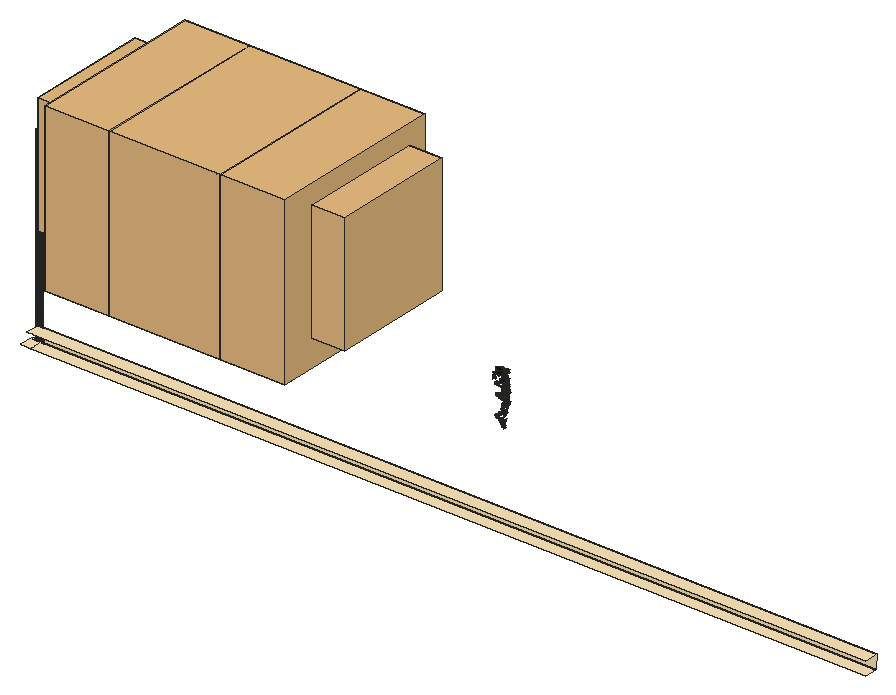
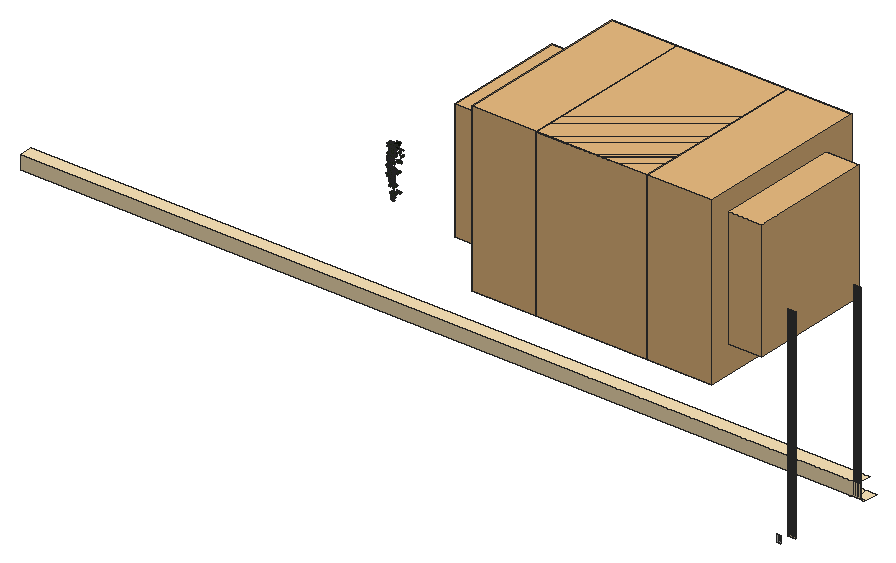
# SketchUp Ruby script. Lengths in inches.
U = 1.inch
M = Sketchup.active_model
def pt(a) = Geom::Point3d.new(a.map { |v| v * U })
def face(e, loops, mat)
  f = e.add_face(loops[0].map { |a| pt(a) })
  loops[1..].each { |l| e.add_face(l.map { |a| pt(a) }).erase! }
  f.material = f.back_material = mat if mat
  f
end
# faces: each face lists its corners as indices into pts; further lists are holes
def faces(e, pts, list, mat = nil) = list.each { |f| face(e, (f[0].is_a?(Array) ? f : [f]).map { |l| l.map { |i| pts[i] } }, mat) }
# xy, xz, yz: faces in a plane at the given z, y or x. An outline is a flat list of corners, or four numbers for a rectangle; further outlines are holes
def ring(l) = l.size == 4 ? [[l[0], l[1]], [l[2], l[1]], [l[2], l[3]], [l[0], l[3]]] : l.each_slice(2).to_a
def flat(e, list, mat, &to3) = list.each { |f| face(e, (f[0].is_a?(Array) ? f : [f]).map { |l| ring(l).map { |u, v| to3.(u, v) } }, mat) }
def xy(e, z, list, mat = nil) = flat(e, list, mat) { |x, y| [x, y, z] }
def xz(e, y, list, mat = nil) = flat(e, list, mat) { |x, z| [x, y, z] }
def yz(e, x, list, mat = nil) = flat(e, list, mat) { |y, z| [x, y, z] }
def lines(e, pts, list) = list.each { |a, b| e.add_line(pt(pts[a]), pt(pts[b])) }
# prism: a flat outline (further loops are holes) pulled along v
def prism(e, loops, v, mat = nil)
  f = face(e, loops, mat); d = Geom::Vector3d.new(v.map { |x| x * U })
  f.pushpull(f.normal.samedirection?(d) ? d.length : -d.length)
end
def box(e, o, s, mat = nil) = prism(e, [[o, [o[0] + s[0], o[1], o[2]], [o[0] + s[0], o[1] + s[1], o[2]], [o[0], o[1] + s[1], o[2]]]], [0, 0, s[2]], mat)
def at(x, y, z, deg = 0) = Geom::Transformation.translation(pt([x, y, z])) * Geom::Transformation.rotation(ORIGIN, Z_AXIS, deg.degrees)
def axes(o, x, y, z) = Geom::Transformation.new([*x, 0, *y, 0, *z, 0, *pt(o).to_a, 1])
def part(name) = M.definitions.add(name)
# library, detail: a bought-in or finely detailed component or shape, given as its bounding box
def library(name, o, s) = part(name).tap { |d| box(d.entities, o, s) }
def detail(e, o, s) = box(e.add_group.entities, o, s)
def put(e, d, t, mat = nil) = e.add_instance(d, t).tap { |i| i.material = mat if mat }
def group(e, t, mat = nil) = e.add_group.tap { |g| g.transformation = t; g.material = mat if mat }.entities
root = M.entities
M.materials.add("1026 AP 7946 SUNNY SIDE UP").color = [254, 231, 186]
M.materials.add("efeu1").color = [18, 25, 13]
M.materials.add("efeu2").color = [43, 57, 29]
c1 = library("Plante \#58",[-0.43,-1.58,0],[20.84,18.06,17.59])
c2 = library("Plant+Philodendron+Scandens",[-5.75,-7.35,0],[25.95,25.95,24.43])
c3 = part("ivyleaf_10")
p = [[0,0.5,-0.03],[-0.0625,2.02,-0.43],[-0.19,2.01,-0.46],[-0.54,1.05,-0.29],[-0.52,0.625,-0.18],[-0.83,0.76,-0.28],
  [-1.16,0.64,-0.33],[-1.15,0.33,-0.24],[-0.77,-0.39,0.02],[-0.3,-0.51,0.16],[0.04,-0.48,0.23],[-0.02,2.01,-0.4375],
  [-0.06,2.01,-0.43],[0.04,-0.49,0.23],[0.67,-0.49,0.14],[1.38,0.36,-0.2],[1.375,0.51,-0.24],[0.81,0.65,-0.19],
  [0.62,0.59,-0.15],[0.6,1.09,-0.28],[0.5,1.23,-0.31]]
faces(c3.entities,p,[[0,1,2,3,4,5,6,7,8,9,10],[11,12,0,13,14,15,16,17,18,19,20]],"efeu2")
c4 = part("ivyleaf_9")
p = [[1.54,2.16,1.25],[1.36,2.04,1.19],[-0.21,0.99,0.68],[-0.71,1.11,0.82],[-0.85,0.86,0.67],[-0.8,0.17,0.21],
  [-0.9,-0.01,0.1],[-0.67,-0.16,-0.02],[-0.08,-0.08,-0.05],[-0.03,-0.6,-0.4],[0.65,-0.88,-0.66],[0.83,-0.6,-0.49],
  [1.29,-0.42,-0.43],[1.8125,-0.07,-0.26],[1.21,0.44,0.15]]
faces(c4.entities,p,[[0,1,2,3,4,5,6,7,8,9,10,11,12,13,14]],"efeu1")
xy(root,246,[[152.978,213.099,30,213.101,29.751,213.101,29.492,213.104,29.53,215.005,29.675,215.002,29.749,215.001,29.764,215.001,30,215,153,215],[29.492,213.104,29.19,213.112,28.983,213.119,28.649,213.135,28.378,213.15,28.108,213.169,27.896,213.185,28.055,215.079,28.117,215.074,28.184,215.069,28.242,215.064,28.294,215.061,28.352,215.057,28.428,215.052,28.493,215.047,28.538,215.045,28.587,215.042,28.673,215.037,28.744,215.033,28.781,215.031,28.822,215.029,28.918,215.025,28.995,215.021,29.025,215.02,29.058,215.019,29.165,215.015,29.246,215.012,29.269,215.011,29.293,215.01,29.416,215.007,29.497,215.005,29.53,215.005],[153,215,30,215.001,29.749,215.001,29.675,215.002,29.53,215.005,29.532,215.104,29.766,215.101,30,215.101,153,215.099],[30,215,29.764,215.001,29.749,215.001,29.675,215.002,29.53,215.005,29.532,215.104,29.766,215.101,30,215.101,153,215.099,153.002,215.099,153,215],[30,215,30,215.001,29.764,215.001],
  [30,215,153,215,30,215.001],[29.497,215.005,29.416,215.007,29.293,215.01,29.269,215.011,29.246,215.012,29.165,215.015,29.058,215.019,29.025,215.02,28.995,215.021,28.918,215.025,28.822,215.029,28.781,215.031,28.744,215.033,28.673,215.037,28.587,215.042,28.538,215.045,28.493,215.047,28.428,215.052,28.352,215.057,28.294,215.061,28.242,215.064,28.184,215.069,28.117,215.074,28.055,215.079,28.064,215.178,28.254,215.163,28.503,215.146,28.752,215.132,29.064,215.118,29.251,215.111,29.532,215.104,29.53,215.005],[29.764,227.001,29.647,227.004,29.749,227.003,29.913,227.001]],"1026 AP 7946 SUNNY SIDE UP")
xy(root,248,[[152.981,213.1,153.004,215.1,30,215.101,29.766,215.101,29.532,215.104,29.251,215.111,29.064,215.118,28.983,213.12,29.19,213.112,29.492,213.105,29.751,213.101,30,213.101]],"1026 AP 7946 SUNNY SIDE UP")
xz(root,215.001,[[29.749,246,29.756,274],[29.756,246,29.764,274]],"1026 AP 7946 SUNNY SIDE UP")
xz(root,215.005,[[29.497,246,29.513,274],[29.513,246,29.529,274]],"1026 AP 7946 SUNNY SIDE UP")
xz(root,227.001,[[29.764,246,29.809,249],[29.809,246,29.913,249]],"1026 AP 7946 SUNNY SIDE UP")
p = [[28.744,215.033,246],[28.781,215.031,246],[28.781,215.031,274],[28.744,215.033,274],[28.822,215.029,246],[28.822,215.029,274],
  [28.918,215.025,246],[28.918,215.025,274],[28.995,215.021,246],[28.995,215.021,274],[29.025,215.02,246],[29.025,215.02,274],
  [29.058,215.019,246],[29.058,215.019,274],[29.165,215.015,246],[29.165,215.015,274],[29.246,215.012,246],[29.246,215.012,274],
  [29.269,215.011,246],[29.269,215.011,274],[29.293,215.01,246],[29.293,215.01,274],[29.416,215.007,246],[29.416,215.007,274],
  [29.497,215.005,246],[29.497,215.005,274],[29.53,215.005,246],[29.675,215.002,246],[29.675,215.002,274],[29.529,215.005,274],
  [29.529,215.005,246],[29.749,215.001,246],[29.749,215.001,274],[29.064,215.118,248],[29.064,215.118,246],[28.752,215.132,246],
  [28.752,215.132,248],[29.251,215.111,248],[29.251,215.111,246],[29.532,215.104,248],[29.532,215.104,246],[29.766,215.101,248],
  [29.766,215.101,246],[153.004,215.1,248],[153.002,215.099,246],[153,215.099,246],[30,215.101,246],[30,215.101,248],
  [28.996,227.042,246],[28.871,227.053,246],[28.871,227.053,276],[28.996,227.042,276],[29.058,227.037,252],[28.902,227.05,252],
  [28.902,227.05,246],[29.058,227.037,246],[29.121,227.032,246],[29.121,227.032,276],[29.247,227.024,246],[29.247,227.024,276],
  [29.215,227.026,252],[29.215,227.026,246],[29.372,227.016,246],[29.372,227.016,276],[29.372,227.016,252],[29.372,227.016,246],
  [29.497,227.011,246],[29.497,227.011,276],[29.529,227.009,252],[29.529,227.009,246],[29.623,227.006,246],[29.623,227.006,276],
  [29.686,227.004,252],[29.686,227.004,246],[29.647,227.004,246],[29.749,227.003,276],[29.749,227.003,246],[29.913,227.001,246],
  [29.913,227.001,276],[29.913,227.001,249],[29.843,227.001,252],[29.843,227.001,246],[30,227,252],[30,227,246],
  [30,227,246],[30,227,276],[28.746,227.066,246],[28.746,227.066,276],[28.746,227.066,252],[28.746,227.066,246],
  [29.477,229.014,246],[29.346,229.021,246],[29.346,229.021,247],[29.477,229.014,247],[29.607,229.008,246],[29.607,229.008,247],
  [29.738,229.003,246],[29.738,229.003,247],[29.869,229.001,246],[29.869,229.001,247],[30,229,246],[30,229,247],
  [29.058,227.037,264],[28.902,227.05,264],[28.902,227.05,252],[29.058,227.037,252],[29.215,227.026,264],[29.215,227.026,252],
  [29.372,227.016,264],[29.372,227.016,252],[29.529,227.009,264],[29.529,227.009,252],[29.686,227.004,264],[29.686,227.004,252],
  [29.843,227.001,264],[29.843,227.001,252],[30,227,264],[30,227,252],[28.746,227.066,264],[28.746,227.066,252],
  [29.808,224.001,249],[29.818,224.001,249],[29.73,224.001,246],[29.73,224.002,246]]
faces(root,p,[[0,1,2,3],[1,4,5,2],[4,6,7,5],[6,8,9,7],[8,10,11,9],[10,12,13,11],[12,14,15,13],[14,16,17,15],
  [16,18,19,17],[18,20,21,19],[20,22,23,21],[22,24,25,23],[26,27,28,29,30],[27,31,32,28],[33,34,35,36],[37,38,34,33],
  [39,40,38,37],[41,42,40,39],[43,44,45,46,42,41,47],[48,49,50,51],[56,48,51,57],[58,56,57,59],[62,58,59,63],[66,62,63,67],
  [70,66,67,71],[74,70,71,75,76],[77,76,75,78,79],[84,77,79,78,85],[49,86,87,50]],"1026 AP 7946 SUNNY SIDE UP")
faces(root,p,[[52,53,54,55],[60,52,55,61],[64,60,61,65],[68,64,65,69],[72,68,69,73],[80,72,73,81],[82,80,81,83],[53,88,89,54],
  [90,91,92,93],[94,90,93,95],[96,94,95,97],[98,96,97,99],[100,98,99,101],[102,103,104,105],[106,102,105,107],[108,106,107,109],
  [110,108,109,111],[112,110,111,113],[114,112,113,115],[116,114,115,117],[103,118,119,104]])
lines(root,p,[[120,121],[122,123]])
put(root,c1,at(36.07,208.25,266.62),"1026 AP 7946 SUNNY SIDE UP")
put(root,c2,at(46.36,209.14,262.56),"1026 AP 7946 SUNNY SIDE UP")
put(root,c2,axes([70.36,209.14,262.56],[-1,0,0],[0,1,0],[0,0,1]),"1026 AP 7946 SUNNY SIDE UP")
put(root,c1,axes([80.64,208.25,266.62],[-1,0,0],[0,1,0],[0,0,1]),"1026 AP 7946 SUNNY SIDE UP")
put(root,c3,axes([97.92,213.16,266.36],[0.01195,0.19185,0.08321],[0.0126,0.07498,-0.20443],[-0.34959,0.00926,-0.00452]),"1026 AP 7946 SUNNY SIDE UP")
put(root,c3,axes([98.22,213.33,266.91],[-0.209,0.12644,0.10282],[-0.12367,0.06066,-0.18786],[-0.2376,-0.14279,0.00734]),"1026 AP 7946 SUNNY SIDE UP")
put(root,c3,axes([98.28,213.28,265.58],[-0.27403,0.01923,-0.121],[0.17853,-0.05393,-0.17101],[-0.07853,-0.18969,0.03346]),"1026 AP 7946 SUNNY SIDE UP")
put(root,c3,axes([98.42,213.13,261.25],[0.24213,-0.01784,-0.13283],[0.21145,0.00255,0.15323],[-0.02001,-0.18888,0.01195]),"1026 AP 7946 SUNNY SIDE UP")
put(root,c3,axes([98.53,213.29,264.14],[0.27977,0.05439,0.07931],[0.12674,0.00695,-0.18497],[-0.0893,0.18027,-0.01405]),"1026 AP 7946 SUNNY SIDE UP")
put(root,c4,axes([98.99,213.21,267.04],[-0.25678,0.03562,0.15458],[-0.24862,-0.00386,-0.16382],[-0.03922,-0.20876,0.02641]),"1026 AP 7946 SUNNY SIDE UP")
put(root,c3,axes([98.72,213.4375,263.99],[-0.02023,0.10774,-0.1576],[-0.03283,-0.14884,-0.11593],[-0.30987,0.00874,0.02257]),"1026 AP 7946 SUNNY SIDE UP")
put(root,c3,axes([98.63,213.4,263.84],[0.10339,-0.05493,-0.17692],[0.23868,-0.0865,0.08542],[-0.17245,-0.15264,0.01216]),"1026 AP 7946 SUNNY SIDE UP")
put(root,c4,axes([98.6,213.07,267.58],[0.17754,0.03197,0.19363],[0.30548,0.02138,-0.11541],[-0.05884,0.20747,-0.01494]),"1026 AP 7946 SUNNY SIDE UP")
put(root,c3,axes([98.83,213.47,267.57],[0.15182,0.1774,0.01825],[0.00379,0.01537,-0.21241],[-0.30216,0.08933,0.00651]),"1026 AP 7946 SUNNY SIDE UP")
put(root,c3,axes([98.9,213.15,260.88],[0.01641,0.1768,0.06511],[0.00077,0.05857,-0.18873],[-0.31614,0.00932,0.00292]),"1026 AP 7946 SUNNY SIDE UP")
put(root,c3,axes([98.89,213.36,266.07],[0.11168,0.1812,0.03792],[0.03798,0.02698,-0.20562],[-0.31036,0.0685,-0.01152]),"1026 AP 7946 SUNNY SIDE UP")
put(root,c3,axes([99.13,213.32,266.61],[-0.24984,0.13472,-0.02037],[0.0099,-0.02434,-0.21342],[-0.23118,-0.14663,0.01288]),"1026 AP 7946 SUNNY SIDE UP")
put(root,c3,axes([99.22,213.45,264.43],[-0.25748,-0.09041,0.03026],[-0.03265,-0.02511,-0.18898],[0.15806,-0.15245,0.01025]),"1026 AP 7946 SUNNY SIDE UP")
put(root,c3,axes([99.26,213.17,262.75],[-0.20879,0.09471,0.0969],[-0.13476,0.04276,-0.16505],[-0.1751,-0.14584,0.01147]),"1026 AP 7946 SUNNY SIDE UP")
put(root,c3,axes([99.125,213.0625,261.79],[0.15268,0.13579,-0.11808],[0.09157,0.09854,0.17555],[0.2845,-0.10459,0.00687]),"1026 AP 7946 SUNNY SIDE UP")
put(root,c3,axes([99.24,213.16,262.92],[-0.21959,0.12081,0.03927],[-0.05627,0.01584,-0.18892],[-0.20602,-0.1331,0.00975]),"1026 AP 7946 SUNNY SIDE UP")
put(root,c3,axes([99.28,213.62,266.06],[-0.31294,0.02243,0.03793],[-0.06817,-0.05289,-0.19018],[-0.01895,-0.18006,0.05782]),"1026 AP 7946 SUNNY SIDE UP")
put(root,c3,axes([99.21,213.58,267.22],[-0.0927,0.18967,-0.005],[-0.00437,-0.00817,-0.21136],[-0.32218,-0.05446,0.00431]),"1026 AP 7946 SUNNY SIDE UP")
put(root,c3,axes([99.24,213.5625,266.91],[-0.22897,-0.1375,-0.03096],[0.06502,0.00005,-0.20417],[0.22886,-0.13758,0.02703]),"1026 AP 7946 SUNNY SIDE UP")
put(root,c3,axes([99.31,213.14,262.35],[-0.2824,0.0536,0.02972],[-0.05164,-0.00651,-0.18648],[-0.08787,-0.16842,0.01407]),"1026 AP 7946 SUNNY SIDE UP")
put(root,c3,axes([99.26,213.1875,260.54],[0.05726,0.17651,0.04323],[-0.05023,0.04362,-0.18778],[-0.30238,0.02618,0.03938]),"1026 AP 7946 SUNNY SIDE UP")
put(root,c3,axes([99.43,213.34,265.14],[-0.22717,-0.08085,0.12232],[-0.14609,-0.07896,-0.1673],[0.18924,-0.15802,0.01768]),"1026 AP 7946 SUNNY SIDE UP")
put(root,c3,axes([99.29,213.52,264.34],[0.29648,-0.01595,-0.03114],[-0.05069,-0.0102,-0.1874],[0.02383,0.17673,-0.01113]),"1026 AP 7946 SUNNY SIDE UP")
put(root,c3,axes([99.45,213.61,264.22],[0.1731,-0.00433,-0.15705],[-0.24903,-0.00162,-0.10918],[0.00194,0.1786,-0.00231]),"1026 AP 7946 SUNNY SIDE UP")
put(root,c3,axes([99.38,213.29,264.99],[-0.09721,0.12519,0.14953],[-0.14359,0.11122,-0.144],[-0.28188,-0.09983,0.02178]),"1026 AP 7946 SUNNY SIDE UP")
put(root,c3,axes([99.34,213.15,260.93],[-0.20264,0.14434,0.00495],[0.01706,0.00476,0.20026],[0.24448,0.11931,-0.00987]),"1026 AP 7946 SUNNY SIDE UP")
put(root,c3,axes([99.28,213.2,260.22],[-0.14191,0.15306,-0.04584],[0.02061,-0.04434,-0.18701],[-0.26995,-0.08385,0.00982]),"1026 AP 7946 SUNNY SIDE UP")
put(root,c3,axes([99.54,213.24,266.15],[-0.14743,0.0292,0.18719],[-0.29796,0.00988,-0.09518],[-0.03724,-0.19464,0.02046]),"1026 AP 7946 SUNNY SIDE UP")
put(root,c3,axes([99.39,213.17,260.48],[-0.3107,-0.01834,0.00171],[0.00004,-0.01854,-0.1962],[0.03128,-0.1821,0.01721]),"1026 AP 7946 SUNNY SIDE UP")
put(root,c3,axes([99.55,213.17,260.14],[-0.1953,0.03857,-0.14149],[-0.19608,0.06787,0.12931],[0.12868,0.16196,-0.0177]),"1026 AP 7946 SUNNY SIDE UP")
put(root,c3,axes([99.38,213.125,263.29],[-0.03087,-0.15106,-0.12006],[0.02786,0.10898,-0.16135],[0.31617,-0.02436,0.00249]),"1026 AP 7946 SUNNY SIDE UP")
put(root,c3,axes([99.36,213.58,265.29],[0.06301,0.14377,-0.11913],[-0.05051,-0.10917,-0.16048],[-0.30643,0.04756,0.00196]),"1026 AP 7946 SUNNY SIDE UP")
put(root,c3,axes([99.49,213.125,262.53],[-0.06118,0.06444,-0.18579],[-0.10151,0.16417,0.08047],[0.29882,0.06897,-0.0107]),"1026 AP 7946 SUNNY SIDE UP")
put(root,c3,axes([99.33,213.42,263.8],[0.02881,0.17787,0.00893],[0.00945,0.00551,-0.19113],[-0.30196,0.01714,-0.00513]),"1026 AP 7946 SUNNY SIDE UP")
put(root,c3,axes([99.38,213.35,266.48],[-0.32401,-0.03464,-0.02888],[0.04945,-0.01256,-0.20702],[0.05514,-0.1923,0.01594]),"1026 AP 7946 SUNNY SIDE UP")
put(root,c4,axes([99.51,212.98,266.375],[0.16688,0.22418,0.01678],[-0.00661,0.01859,-0.25513],[-0.35323,0.10556,0.0127]),"1026 AP 7946 SUNNY SIDE UP")
put(root,c3,axes([99.39,213.64,265.25],[0.06844,0.10736,0.15478],[0.07604,0.13604,-0.12081],[-0.29411,0.06016,0.00478]),"1026 AP 7946 SUNNY SIDE UP")
put(root,c3,axes([99.6,213.42,267.67],[-0.1306,-0.1552,0.1188],[-0.06394,-0.10716,-0.18652],[0.31954,-0.08487,0.01123]),"1026 AP 7946 SUNNY SIDE UP")
put(root,c3,axes([99.5625,213.2,265.4],[-0.24737,-0.13133,-0.0181],[0.03601,-0.00091,-0.20942],[0.22151,-0.14651,0.01383]),"1026 AP 7946 SUNNY SIDE UP")
put(root,c3,axes([99.76,213.48,262.78],[-0.03155,0.0469,0.18196],[-0.28421,0.04699,-0.03295],[-0.0906,-0.16376,0.03999]),"1026 AP 7946 SUNNY SIDE UP")
put(root,c3,axes([99.5625,213.19,260.85],[0.04999,-0.10427,0.14964],[-0.05743,0.13705,0.11787],[-0.29229,-0.04476,0.00243]),"1026 AP 7946 SUNNY SIDE UP")
put(root,c3,axes([99.62,213.37,262.88],[0.04293,0.00088,0.18984],[-0.11223,0.16624,0.01153],[-0.2793,-0.06667,0.02455]),"1026 AP 7946 SUNNY SIDE UP")
put(root,c3,axes([99.78,213.34,263.72],[0.08987,0.00627,-0.19426],[-0.28059,-0.07675,-0.05551],[-0.12787,0.17282,-0.01471]),"1026 AP 7946 SUNNY SIDE UP")
put(root,c3,axes([99.57,213.1875,262.01],[0.00467,0.14653,-0.10508],[0.00114,-0.10008,-0.15828],[-0.3012,0.00189,-0.00223]),"1026 AP 7946 SUNNY SIDE UP")
put(root,c3,axes([99.54,213.55,265.79],[0.32011,-0.00023,0.02372],[0.0374,-0.01862,-0.20117],[0.00407,0.18895,-0.01714]),"1026 AP 7946 SUNNY SIDE UP")
put(root,c4,axes([99.71,212.96,265.52],[0.09311,0.17322,0.17021],[-0.04204,0.17297,-0.17698],[-0.37297,0.02374,0.06244]),"1026 AP 7946 SUNNY SIDE UP")
put(root,c3,axes([99.66,213.16,265.65],[-0.20242,-0.14868,-0.002],[0.01736,-0.00829,-0.20367],[0.25179,-0.11895,0.01243]),"1026 AP 7946 SUNNY SIDE UP")
put(root,c3,axes([99.6,213.12,261.875],[0.02757,-0.03956,0.19236],[0.00436,0.18092,0.04481],[-0.31314,-0.00097,0.01756]),"1026 AP 7946 SUNNY SIDE UP")
put(root,c3,axes([99.64,213.61,264.3],[-0.08999,0.16367,-0.05113],[-0.02158,-0.05586,-0.18248],[-0.28965,-0.04669,0.02948]),"1026 AP 7946 SUNNY SIDE UP")
put(root,c3,axes([99.66,213.5,266.18],[0.27478,-0.10868,-0.02402],[-0.03177,0.00983,-0.20858],[0.18521,0.16293,-0.00014]),"1026 AP 7946 SUNNY SIDE UP")
put(root,c3,axes([99.59,213.15,264.22],[0.11642,0.17369,0.00614],[0.01286,0.00074,-0.19978],[-0.29463,0.06866,-0.00629]),"1026 AP 7946 SUNNY SIDE UP")
put(root,c3,axes([99.64,213.49,265.52],[-0.29636,-0.07513,-0.04489],[0.08741,-0.01794,-0.20004],[0.11601,-0.17842,0.03606]),"1026 AP 7946 SUNNY SIDE UP")
put(root,c3,axes([99.67,213.47,265.19],[-0.29428,0.07166,-0.03821],[0.03147,-0.04909,-0.19744],[-0.13295,-0.17025,0.03785]),"1026 AP 7946 SUNNY SIDE UP")
put(root,c3,axes([99.79,213.125,263.27],[0.16843,-0.1344,-0.1236],[-0.1291,0.08498,-0.17741],[0.26952,0.1247,-0.00774]),"1026 AP 7946 SUNNY SIDE UP")
put(root,c3,axes([99.63,213.49,266.4375],[-0.16116,0.15069,-0.09103],[0.05796,-0.08104,-0.19131],[-0.28963,-0.10007,0.01237]),"1026 AP 7946 SUNNY SIDE UP")
put(root,c3,axes([99.72,213.5,266.02],[-0.09746,0.15812,0.1028],[-0.06366,0.0863,-0.17881],[-0.30568,-0.06839,0.00446]),"1026 AP 7946 SUNNY SIDE UP")
put(root,c3,axes([99.69,213.48,266.79],[-0.15805,0.17613,-0.02982],[-0.00673,-0.03602,-0.2127],[-0.30326,-0.09099,0.02026]),"1026 AP 7946 SUNNY SIDE UP")
put(root,c3,axes([99.7,213.22,266.16],[0.03305,0.15417,-0.1198],[-0.05875,-0.10979,-0.16694],[-0.32005,0.03607,0.01828]),"1026 AP 7946 SUNNY SIDE UP")
put(root,c3,axes([99.63,213.57,265.62],[0.28073,-0.07597,0.05242],[0.06635,-0.03421,-0.19471],[0.13935,0.16933,-0.01289]),"1026 AP 7946 SUNNY SIDE UP")
put(root,c3,axes([99.6875,213.5,265.79],[-0.11431,0.17426,-0.03499],[0.00561,-0.03614,-0.20024],[-0.30166,-0.06671,0.00954]),"1026 AP 7946 SUNNY SIDE UP")
put(root,c3,axes([99.68,213.46,264.36],[0.01177,-0.06871,0.18563],[0.02607,0.17403,0.07522],[-0.31694,0.01176,0.01308]),"1026 AP 7946 SUNNY SIDE UP")
put(root,c3,axes([99.7,213.42,267.26],[-0.03586,-0.16954,0.11817],[0.01268,0.11247,0.18439],[-0.34526,0.02174,-0.0055]),"1026 AP 7946 SUNNY SIDE UP")
put(root,c3,axes([99.83,213.07,265.48],[0.07736,-0.01682,-0.20619],[-0.0596,0.19364,-0.02432],[0.32235,0.03984,0.04499]),"1026 AP 7946 SUNNY SIDE UP")
put(root,c3,axes([99.7,213.26,265.15],[0.17908,0.15321,-0.00576],[0.00752,-0.01199,-0.199],[-0.26028,0.10507,-0.00971]),"1026 AP 7946 SUNNY SIDE UP")
put(root,c3,axes([99.76,213.54,265.47],[-0.08997,0.15189,0.11063],[0.06978,-0.09291,0.17077],[0.30202,0.06671,-0.0065]),"1026 AP 7946 SUNNY SIDE UP")
put(root,c3,axes([99.74,213.53,264.77],[0.2193,0.12481,-0.03483],[-0.03012,-0.03073,-0.19246],[-0.21759,0.13005,-0.00846]),"1026 AP 7946 SUNNY SIDE UP")
put(root,c3,axes([99.72,213.5,264.7],[0.09148,-0.1791,-0.0247],[0.01813,-0.01843,0.1999],[-0.30552,-0.05472,0.00447]),"1026 AP 7946 SUNNY SIDE UP")
put(root,c3,axes([99.8,213.55,264.87],[0.11232,-0.16931,0.04125],[0.01803,-0.03958,-0.19511],[0.29506,0.06687,-0.00378]),"1026 AP 7946 SUNNY SIDE UP")
put(root,c3,axes([99.76,213.49,266.46],[0.02711,0.1934,-0.01399],[0.00117,-0.0157,-0.20797],[-0.32938,0.01586,-0.00189]),"1026 AP 7946 SUNNY SIDE UP")
put(root,c3,axes([99.71,213.55,263.47],[-0.25136,0.00704,-0.10184],[0.15376,-0.04519,-0.15501],[-0.05124,-0.17014,0.03441]),"1026 AP 7946 SUNNY SIDE UP")
put(root,c3,axes([99.87,213.0625,262.46],[-0.06081,0.09486,0.16919],[-0.12337,0.13932,-0.10606],[-0.28559,-0.08038,0.00979]),"1026 AP 7946 SUNNY SIDE UP")
put(root,c3,axes([99.76,213.49,264.19],[-0.09631,0.16263,-0.06238],[0.02855,-0.05808,-0.18518],[-0.2931,-0.0591,0.00246]),"1026 AP 7946 SUNNY SIDE UP")
put(root,c3,axes([99.95,213.1,264.99],[0.15177,0.01964,0.18042],[-0.22537,0.12631,0.0615],[-0.17864,-0.14267,0.0757]),"1026 AP 7946 SUNNY SIDE UP")
put(root,c3,axes([99.82,213.2,263.61],[0.05409,-0.11941,0.1398],[-0.05352,0.12833,0.13408],[-0.29755,-0.04479,0.00129]),"1026 AP 7946 SUNNY SIDE UP")
